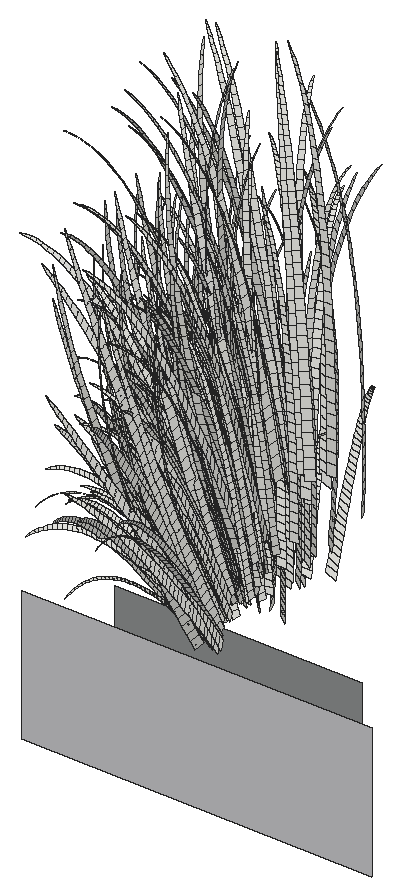
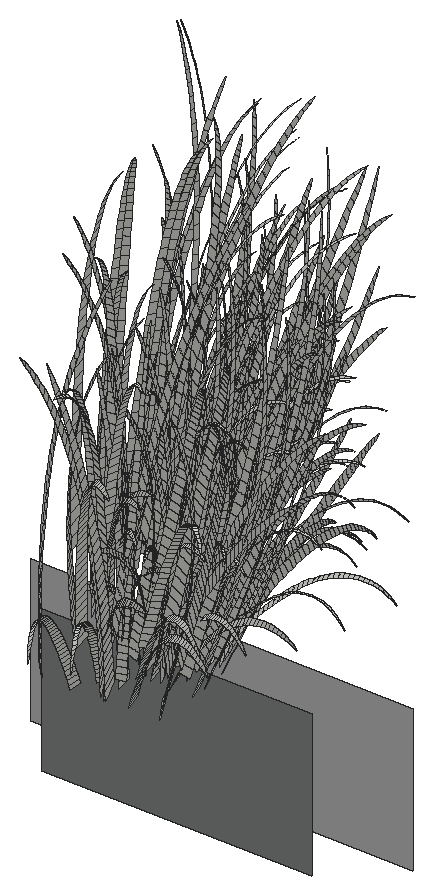
# SketchUp Ruby script. Lengths in inches.
U = 1.inch
M = Sketchup.active_model
def pt(a) = Geom::Point3d.new(a.map { |v| v * U })
def face(e, loops, mat)
  f = e.add_face(loops[0].map { |a| pt(a) })
  loops[1..].each { |l| e.add_face(l.map { |a| pt(a) }).erase! }
  f.material = f.back_material = mat if mat
  f
end
# faces: each face lists its corners as indices into pts; further lists are holes
def faces(e, pts, list, mat = nil) = list.each { |f| face(e, (f[0].is_a?(Array) ? f : [f]).map { |l| l.map { |i| pts[i] } }, mat) }
# xy, xz, yz: faces in a plane at the given z, y or x. An outline is a flat list of corners, or four numbers for a rectangle; further outlines are holes
def ring(l) = l.size == 4 ? [[l[0], l[1]], [l[2], l[1]], [l[2], l[3]], [l[0], l[3]]] : l.each_slice(2).to_a
def flat(e, list, mat, &to3) = list.each { |f| face(e, (f[0].is_a?(Array) ? f : [f]).map { |l| ring(l).map { |u, v| to3.(u, v) } }, mat) }
def xy(e, z, list, mat = nil) = flat(e, list, mat) { |x, y| [x, y, z] }
def xz(e, y, list, mat = nil) = flat(e, list, mat) { |x, z| [x, y, z] }
def yz(e, x, list, mat = nil) = flat(e, list, mat) { |y, z| [x, y, z] }
def lines(e, pts, list) = list.each { |a, b| e.add_line(pt(pts[a]), pt(pts[b])) }
# prism: a flat outline (further loops are holes) pulled along v
def prism(e, loops, v, mat = nil)
  f = face(e, loops, mat); d = Geom::Vector3d.new(v.map { |x| x * U })
  f.pushpull(f.normal.samedirection?(d) ? d.length : -d.length)
end
def box(e, o, s, mat = nil) = prism(e, [[o, [o[0] + s[0], o[1], o[2]], [o[0] + s[0], o[1] + s[1], o[2]], [o[0], o[1] + s[1], o[2]]]], [0, 0, s[2]], mat)
def at(x, y, z, deg = 0) = Geom::Transformation.translation(pt([x, y, z])) * Geom::Transformation.rotation(ORIGIN, Z_AXIS, deg.degrees)
def axes(o, x, y, z) = Geom::Transformation.new([*x, 0, *y, 0, *z, 0, *pt(o).to_a, 1])
def part(name) = M.definitions.add(name)
# library, detail: a bought-in or finely detailed component or shape, given as its bounding box
def library(name, o, s) = part(name).tap { |d| box(d.entities, o, s) }
def detail(e, o, s) = box(e.add_group.entities, o, s)
def put(e, d, t, mat = nil) = e.add_instance(d, t).tap { |i| i.material = mat if mat }
def group(e, t, mat = nil) = e.add_group.tap { |g| g.transformation = t; g.material = mat if mat }.entities
root = M.entities
M.materials.add("[Blacktop Old 02]").color = [143, 145, 145]
M.materials.add("[Polished Concrete New]").color = [200, 200, 203]
c1 = part("fur_instance\#8")
p = [[-0.25,1.49,0.03],[0.25,-1.49,-0.03],[0.44,-1.47,1.51],[-0.05,1.47,1.57],[0.65,-1.44,3.05],[0.16,1.45,3.11],
  [0.86,-1.42,4.59],[0.38,1.44,4.65],[1.1,-1.39,6.13],[0.62,1.43,6.18],[1.34,-1.35,7.66],[0.875,1.42,7.72],
  [1.6,-1.32,9.19],[1.14,1.41,9.25],[1.88,-1.28,10.72],[1.43,1.41,10.78],[2.18,-1.24,12.25],[1.73,1.41,12.3],
  [2.49,-1.19,13.77],[2.05,1.41,13.82],[2.83,-1.15,15.29],[2.4,1.41,15.34],[3.18,-1.09,16.8],[2.76,1.42,16.85],
  [3.56,-1.03,18.31],[3.14,1.43,18.35],[3.96,-0.97,19.81],[3.55,1.44,19.85],[4.38,-0.91,21.3],[3.99,1.46,21.35],
  [4.84,-0.83,22.78],[4.45,1.48,22.83],[5.32,-0.76,24.26],[4.93,1.51,24.31],[5.82,-0.67,25.73],[5.45,1.54,25.77],
  [6.36,-0.59,27.18],[6,1.57,27.23],[6.93,-0.49,28.625],[6.58,1.61,28.67],[7.54,-0.39,30.05],[7.19,1.66,30.1],
  [8.18,-0.28,31.47],[7.84,1.71,31.51],[8.85,-0.16,32.86],[8.53,1.77,32.9],[9.57,-0.04,34.24],[9.25,1.83,34.27],
  [10.32,0.09,35.59],[10.02,1.9,35.625],[11.12,0.23,36.92],[10.82,1.97,36.95],[11.95,0.38,38.22],[11.67,2.06,38.25],
  [12.84,0.54,39.49],[12.57,2.14,39.52],[13.76,0.71,40.73],[13.51,2.24,40.76],[14.73,0.89,41.93],[14.49,2.34,41.95],
  [15.75,1.08,43.09],[15.52,2.45,43.11],[16.82,1.28,44.2],[16.6,2.5625,44.23],[17.93,1.5,45.27],[17.73,2.68,45.29],
  [19.08,1.73,46.28],[18.9,2.81,46.3],[20.29,1.97,47.24],[20.125,2.93,47.26],[21.53,2.22,48.13],[21.39,3.0625,48.15],
  [22.82,2.5,48.96],[22.7,3.1875,48.98],[24.14,2.8125,49.72],[24.06,3.3,49.73],[25.48,3.27,50.41]]
faces(c1.entities,p,[[0,1,2,3],[3,2,4,5],[5,4,6,7],[7,6,8,9],[9,8,10,11],[11,10,12,13],[13,12,14,15],[15,14,16,17],
  [17,16,18,19],[19,18,20,21],[21,20,22,23],[23,22,24,25],[25,24,26,27],[27,26,28,29],[29,28,30,31],[31,30,32,33],
  [33,32,34,35],[35,34,36,37],[37,36,38,39],[39,38,40,41],[41,40,42,43],[43,42,44,45],[45,44,46,47],[47,46,48,49],
  [49,48,50,51],[51,50,52,53],[53,52,54,55],[55,54,56,57],[57,56,58,59],[59,58,60,61],[61,60,62,63],[63,62,64,65],
  [65,64,66,67],[67,66,68,69],[69,68,70,71],[71,70,72,73],[73,72,74,75],[75,74,76]])
xz(root,47.02,[[415.52,0,442.8125,10.375]],"[Polished Concrete New]")
xz(root,51.02,[[419.51,0,438.8125,10.375]],"[Blacktop Old 02]")
put(root,c1,axes([426.79,51.39,16.74],[-0.23554,0.05296,-0.19778],[0.0198,-0.2043,-0.19606],[-0.09324,-0.11985,0.49597]))
put(root,c1,axes([425.38,56.38,16.61],[-0.04995,0.23864,-0.11124],[-0.21419,-0.02204,-0.24055],[-0.12191,-0.01612,0.49664]))
put(root,c1,axes([426.6,51.125,11.45],[-0.11039,-0.00414,-0.3495],[0.07669,-0.1786,0.00651],[-0.14786,-0.06719,0.2791]))
put(root,c1,axes([427.18,49.875,11.47],[-0.13594,0.15084,-0.11164],[-0.0609,-0.07291,-0.33491],[-0.13519,-0.09407,0.27953]))
put(root,c1,axes([426.68,55.02,12.58],[-0.1218,-0.13361,-0.0921],[0.11484,-0.14709,0.28095],[-0.12602,0.02393,0.36414]))
put(root,c1,axes([427.19,53.87,10.88],[-0.1289,0.01316,-0.29885],[-0.02366,-0.17656,0.13341],[-0.13753,0.03975,0.27153]))
put(root,c1,axes([424.89,53.64,11.67],[0.13391,-0.00422,0.37894],[-0.02725,0.21287,-0.08205],[-0.17659,-0.01268,0.31548]))
put(root,c1,axes([426.69,57.03,14.76],[-0.09952,0.18231,-0.31022],[-0.16857,-0.11721,-0.10121],[-0.1255,0.04853,0.40556]))
put(root,c1,axes([424.78,54.78,11.59],[0.14067,-0.04522,0.3848],[0.02544,0.20918,-0.05629],[-0.17357,0.01812,0.31957]))
put(root,c1,axes([425.36,55.57,13.76],[0.05993,0.19956,0.02934],[-0.16765,0.09615,-0.32784],[-0.14862,0.00196,0.40149]))
put(root,c1,axes([426.36,56.78,16.92],[-0.0789,0.22714,-0.18379],[-0.20548,-0.06456,-0.18143],[-0.11262,0.00359,0.48952]))
put(root,c1,axes([427.34,57.21,11.14],[-0.14657,0.06865,-0.32949],[-0.09952,-0.16829,0.15169],[-0.11649,0.08935,0.30613]))
put(root,c1,axes([427.57,50.6,12.74],[-0.14992,0.10635,-0.20855],[-0.03569,-0.13875,-0.18978],[-0.12006,-0.06524,0.33426]))
put(root,c1,axes([427.57,52.03,12.61],[-0.13947,0.07457,-0.26376],[-0.03048,-0.16347,-0.05841],[-0.12421,-0.01975,0.3263]))
put(root,c1,axes([427.6,50.76,11.21],[-0.11214,0.07357,-0.29467],[-0.00419,-0.1506,-0.10442],[-0.13991,-0.03543,0.25192]))
put(root,c1,axes([426.66,54.32,19.19],[-0.16722,-0.14584,-0.14657],[0.18274,-0.19209,0.09427],[-0.0816,-0.06233,0.55718]))
put(root,c1,axes([427.44,54.59,11.82],[-0.12578,-0.12091,-0.0564],[0.08033,-0.12818,0.33188],[-0.12725,0.06361,0.28183]))
put(root,c1,axes([427.75,56.86,19.51],[-0.24661,-0.01011,-0.12308],[0.03558,-0.24626,0.10561],[-0.06805,-0.01098,0.55498]))
put(root,c1,axes([425.25,57.28,11.43],[0.15352,0.06911,0.26676],[-0.03494,0.20117,-0.28887],[-0.16523,0.04776,0.32623]))
put(root,c1,axes([425.19,55.28,12.72],[0.10956,-0.18152,0.25882],[0.13509,0.11782,0.19082],[-0.14519,0.00192,0.39222]))
put(root,c1,axes([426.18,53.23,12.1],[0.07012,-0.18381,0.20265],[0.10518,0.07075,0.29594],[-0.16336,-0.01173,0.29184]))
put(root,c1,axes([426.59,53.01,16.52],[-0.04128,-0.19919,-0.10991],[0.2038,-0.09544,0.23105],[-0.11682,-0.05581,0.46862]))
put(root,c1,axes([427.86,55.84,12.125],[-0.12441,0.08913,-0.33358],[-0.11522,-0.1494,0.09624],[-0.1115,0.08552,0.29301]))
put(root,c1,axes([425.76,51.14,10.98],[0.13283,-0.0342,0.36955],[-0.05695,0.18902,0.06859],[-0.15898,-0.07225,0.3001]))
put(root,c1,axes([426.07,51.01,11.44],[0.11177,0.01694,0.37048],[-0.08915,0.18926,-0.03147],[-0.15727,-0.07147,0.29687]))
put(root,c1,axes([426.59,51.64,11.96],[0.07273,0.09595,0.27862],[-0.10249,0.16133,-0.212],[-0.15668,-0.03967,0.28211]))
put(root,c1,axes([425.11,52.54,12.71],[0.16226,-0.13696,0.26442],[0.06401,0.16282,0.19515],[-0.14822,-0.05035,0.39313]))
put(root,c1,axes([427.95,52.64,17.74],[-0.19486,-0.07064,-0.15993],[0.11436,-0.20339,0.01183],[-0.07048,-0.06892,0.50496]))
put(root,c1,axes([427.38,58.9,16.65],[-0.12046,-0.19753,0.07695],[0.20061,-0.12871,0.24478],[-0.08711,0.03599,0.49657]))
put(root,c1,axes([428.29,55.15,15.83],[-0.16212,0.13096,-0.2268],[-0.11678,-0.16208,0.00347],[-0.08971,0.01858,0.43465]))
put(root,c1,axes([428.23,53.08,11.33],[-0.11086,0.06293,-0.29386],[-0.07533,-0.1452,0.07106],[-0.11428,0.05713,0.25311]))
put(root,c1,axes([428.16,49.42,10.79],[-0.09839,0.14314,-0.01192],[-0.08354,-0.02419,-0.30566],[-0.11714,-0.08151,0.24221]))
put(root,c1,axes([427.55,52.27,11.29],[-0.01321,-0.17005,0.06481],[0.1141,-0.02557,0.30569],[-0.13946,0.01456,0.25678]))
put(root,c1,axes([428.66,53.23,15.55],[-0.18243,0.01895,-0.19563],[-0.00133,-0.1948,0.08688],[-0.09334,0.00298,0.40574]))
put(root,c1,axes([428.14,60.79,16.22],[-0.18658,0.14503,-0.30144],[-0.1645,-0.17028,0.18908],[-0.06369,0.10062,0.4514]))
put(root,c1,axes([428.72,48.89,11.48],[-0.12873,0.10197,-0.18861],[-0.01018,-0.10343,-0.24101],[-0.11719,-0.08155,0.24232]))
put(root,c1,axes([428.53,51.95,13.6],[-0.16023,0.03354,-0.19126],[-0.00898,-0.17162,0.02853],[-0.08895,-0.01176,0.36236]))
put(root,c1,axes([428.06,52.97,12.5],[-0.0676,0.15738,-0.2157],[-0.13135,-0.07732,-0.14677],[-0.1112,0.02111,0.32133]))
put(root,c1,axes([428.49,50.69,14.9375],[-0.1494,0.14445,-0.05993],[-0.10862,-0.10225,-0.21391],[-0.08642,-0.08137,0.39881]))
put(root,c1,axes([425.98,52.1875,13.6],[0.16036,-0.12824,0.26431],[0.05712,0.1633,0.18167],[-0.14465,-0.04914,0.38366]))
put(root,c1,axes([428,52.12,15.66],[-0.08516,-0.14739,-0.15062],[0.16457,-0.13044,0.17116],[-0.1041,-0.04973,0.41758]))
put(root,c1,axes([426.39,52.24,12.83],[0.12489,0.06673,0.27563],[-0.09958,0.18305,-0.12082],[-0.13573,-0.04611,0.36]))
put(root,c1,axes([428.82,48.28,11.89],[-0.15935,0.03269,-0.28558],[0.09029,-0.13292,-0.22683],[-0.09601,-0.14239,0.28508]))
put(root,c1,axes([428.82,48.72,11.18],[-0.14081,0.09765,-0.1356],[-0.01218,-0.08683,-0.27326],[-0.10036,-0.10168,0.23982]))
put(root,c1,axes([428.96,50.15,15.48],[-0.18347,0.1171,-0.07334],[-0.07461,-0.13251,-0.22152],[-0.07812,-0.10043,0.41558]))
put(root,c1,axes([428.84,48.58,11.68],[-0.15082,0.11254,-0.07354],[-0.05779,-0.09193,-0.25822],[-0.08893,-0.09949,0.31347]))
put(root,c1,axes([428.79,50.79,13.44],[-0.15052,-0.00251,-0.18515],[0.03159,-0.16716,0.03488],[-0.08794,-0.02622,0.34898]))
put(root,c1,axes([428.83,50.58,14.92],[-0.149,-0.04647,-0.21352],[0.09287,-0.17245,0.02054],[-0.09229,-0.06322,0.38876]))
put(root,c1,axes([428.96,53.85,16.78],[-0.20159,0.0718,-0.13723],[-0.04865,-0.19336,0.01671],[-0.06325,-0.01861,0.46524]))
put(root,c1,axes([428.85,53.46,11.04],[-0.13656,-0.07352,-0.06681],[0.04427,-0.12761,0.28622],[-0.09439,0.0724,0.24805]))
put(root,c1,axes([428.77,58.21,17.75],[-0.1589,0.17803,-0.2479],[-0.17756,-0.14881,0.0508],[-0.06832,0.04712,0.49383]))
put(root,c1,axes([428.87,52.13,12],[-0.10384,0.1021,-0.23208],[-0.0841,-0.12138,-0.04288],[-0.10059,0.0191,0.29067]))
put(root,c1,axes([428.34,48.34,12.01],[-0.09966,0.12678,0.30336],[-0.19172,0.0268,-0.26785],[-0.07616,-0.17634,0.31506]))
put(root,c1,axes([428.51,52.76,14.16],[-0.10618,-0.13262,-0.04878],[0.13367,-0.1263,0.19427],[-0.08735,0.00279,0.37967]))
put(root,c1,axes([428.99,57.38,11.26],[-0.17971,0.05049,-0.21333],[-0.08082,-0.15328,0.27859],[-0.06056,0.11282,0.29972]))
put(root,c1,axes([427.36,52.25,10.78],[0.10833,0.05099,0.24664],[-0.03776,0.16401,-0.19126],[-0.1393,0.01454,0.25647]))
put(root,c1,axes([428.48,54.85,20.375],[-0.09372,-0.20637,-0.07363],[0.22677,-0.12712,0.15354],[-0.08199,-0.04812,0.55353]))
put(root,c1,axes([427.59,50.48,12.19],[0.05365,-0.16969,-0.03778],[0.13986,-0.00916,0.27148],[-0.1167,-0.06341,0.32492]))
put(root,c1,axes([429.32,53.85,12.44],[-0.13323,0.08202,-0.23675],[-0.08835,-0.14174,0.08371],[-0.08237,0.05187,0.31467]))
put(root,c1,axes([429.05,48.83,11.85],[-0.10552,0.13111,0.03774],[-0.1075,-0.03434,-0.24755],[-0.08294,-0.09279,0.29236]))
put(root,c1,axes([429.6,48.91,15.38],[-0.23362,0.09843,0.07428],[-0.08627,-0.11761,-0.36241],[-0.04076,-0.18596,0.42692]))
put(root,c1,axes([428.79,49.16,11.5625],[-0.05906,0.14196,0.06951],[-0.12604,0.00717,-0.23329],[-0.09379,-0.07416,0.28621]))
put(root,c1,axes([426.9,53.26,13.26],[0.15491,-0.05585,0.29054],[0.02871,0.18789,-0.02061],[-0.13151,0.00174,0.35528]))
put(root,c1,axes([429.51,51.98,14.7],[-0.13836,0.10656,-0.19014],[-0.08729,-0.13946,-0.02631],[-0.08371,0.00267,0.36384]))
put(root,c1,axes([427.49,49.11,10.74],[0.08197,-0.14846,-0.17255],[0.1435,-0.03613,0.3122],[-0.11735,-0.1189,0.28043]))
put(root,c1,axes([429.62,51.47,18.39],[-0.2227,-0.02851,-0.13015],[0.07795,-0.20389,-0.10631],[-0.04666,-0.10194,0.51151]))
put(root,c1,axes([428.39,50.93,12.49],[0.03066,0.14936,0.05869],[-0.12804,0.07175,-0.24213],[-0.11455,-0.01821,0.30092]))
put(root,c1,axes([429.01,49.93,11.92],[-0.05395,-0.10392,-0.15053],[0.10796,-0.10426,0.17042],[-0.10255,-0.03484,0.272]))
put(root,c1,axes([428.76,51,16.38],[-0.03053,0.18634,0.11663],[-0.19498,0.03215,-0.20672],[-0.09234,-0.08694,0.42611]))
put(root,c1,axes([428.01,56.42,13.39],[0.01665,-0.19186,0.25247],[0.18867,0.0288,0.15737],[-0.09759,0.06145,0.3728]))
put(root,c1,axes([429.6,48.2,12.62],[-0.17727,0.00029,-0.20455],[0.08516,-0.1353,-0.21935],[-0.05731,-0.14134,0.34686]))
put(root,c1,axes([429.36,48.68,12.49],[-0.10062,-0.049,-0.26041],[0.12035,-0.13237,-0.01381],[-0.08638,-0.09663,0.30447]))
put(root,c1,axes([429.01,50.15,14.97],[-0.076,0.1669,0.09562],[-0.17144,-0.01335,-0.19918],[-0.07397,-0.09509,0.39348]))
put(root,c1,axes([429.47,55.02,20.71],[-0.19599,0.17659,-0.04249],[-0.16606,-0.16516,-0.03794],[-0.03174,-0.0516,0.57661]))
put(root,c1,axes([429.33,51.97,15.31],[-0.14595,-0.08896,-0.08701],[0.11069,-0.159,0.08949],[-0.05969,-0.02587,0.41282]))
put(root,c1,axes([429.33,50.94,15.48],[-0.13003,0.1505,-0.04051],[-0.13515,-0.09639,-0.12681],[-0.0585,-0.05721,0.41915]))
put(root,c1,axes([428.24,53.16,19.38],[-0.01349,0.22403,0.09768],[-0.24396,0.034,-0.14422],[-0.06912,-0.0865,0.54108]))
put(root,c1,axes([429.66,50.28,13.09],[-0.12457,-0.03797,-0.15408],[0.05979,-0.14532,0.07008],[-0.07901,-0.02356,0.31353]))
put(root,c1,axes([429.48,55.42,20.55],[-0.19695,0.1732,-0.04859],[-0.16287,-0.16855,-0.01576],[-0.02749,-0.04327,0.57313]))
put(root,c1,axes([429.3,48.07,13.0625],[-0.15374,0.14658,0.25603],[-0.19784,-0.04817,-0.27014],[-0.04101,-0.18709,0.42951]))
put(root,c1,axes([429.32,53.8,19.28],[-0.20007,-0.1011,-0.05198],[0.13259,-0.20105,0.02025],[-0.03025,-0.05245,0.53866]))
put(root,c1,axes([427.7,49.47,10.74],[0.13307,-0.06357,0.27984],[-0.03809,0.14212,0.17121],[-0.12562,-0.08741,0.25976]))
put(root,c1,axes([429.82,53.67,20.4],[-0.23914,-0.05106,-0.06078],[0.08551,-0.22855,-0.0252],[-0.02809,-0.06875,0.5682]))
put(root,c1,axes([427.47,54.33,16.17],[0.12687,0.1431,0.11306],[-0.15006,0.15928,-0.20805],[-0.10892,-0.0144,0.44372]))
put(root,c1,axes([428.26,52,10.79],[0.06974,-0.11239,0.27242],[0.09117,0.10684,0.0892],[-0.12045,0.03482,0.23783]))
put(root,c1,axes([427.44,53.55,12.375],[0.12819,-0.10555,0.27193],[0.08655,0.15023,0.02614],[-0.11644,0.02211,0.33646]))
put(root,c1,axes([426.89,55.5,13.38],[0.17949,0.03208,0.20009],[-0.02216,0.19765,-0.22548],[-0.11594,0.04484,0.37468]))
put(root,c1,axes([428.58,54.41,15.93],[0.00664,0.20286,-0.1262],[-0.19518,0.01818,-0.18229],[-0.08769,0.01816,0.42485]))
put(root,c1,axes([429.57,48.37,11.35],[-0.0986,0.1202,0.03133],[-0.09749,-0.03341,-0.22837],[-0.07635,-0.08541,0.26912]))
put(root,c1,axes([430.06,56.61,13.21],[-0.18808,0.05687,-0.16759],[-0.06647,-0.17012,0.23097],[-0.05108,0.08069,0.36201]))
put(root,c1,axes([429.36,48.13,10.95],[-0.08725,-0.02366,-0.29756],[0.12591,-0.11202,-0.06714],[-0.0803,-0.1191,0.23844]))
put(root,c1,axes([429.89,48.21,11.93],[-0.15103,0.03829,-0.1475],[0.02836,-0.11444,-0.19385],[-0.06472,-0.10394,0.28282]))
put(root,c1,axes([427.19,49.96,12.54],[0.17403,-0.06722,0.24815],[-0.01797,0.16553,0.179],[-0.11789,-0.09322,0.35975]))
put(root,c1,axes([428.86,47.625,10.93],[-0.07738,0.12181,0.42116],[-0.24475,0.02807,-0.19007],[-0.04925,-0.2161,0.35893]))
put(root,c1,axes([427.55,55.9375,13.65],[0.149,0.11824,0.07488],[-0.1012,0.16059,-0.29075],[-0.11547,0.04466,0.37315]))
put(root,c1,axes([430.08,47.65,11.93],[-0.19758,0.0885,0.1271],[-0.09447,-0.05952,-0.37318],[-0.04202,-0.18438,0.30623]))
put(root,c1,axes([428.43,50.7,11.09],[0.09888,-0.02928,0.28041],[-0.00291,0.15131,-0.01175],[-0.12783,-0.00918,0.22836]))
put(root,c1,axes([428.21,57.21,12.21],[0.03058,-0.16302,0.35291],[0.18885,0.05742,0.07777],[-0.09099,0.10522,0.30707]))
put(root,c1,axes([428.5625,49.52,12.4],[0.04667,0.10587,0.22641],[-0.14224,0.11026,-0.13144],[-0.10087,-0.07976,0.30781]))
put(root,c1,axes([428.95,52.48,12.72],[-0.01787,-0.16163,0.13786],[0.14541,-0.01364,0.20157],[-0.09392,0.03632,0.30351]))
put(root,c1,axes([429.45,49.06,15.16],[-0.12023,0.16893,0.15811],[-0.19192,-0.04724,-0.20175],[-0.05017,-0.13536,0.45159]))
put(root,c1,axes([429.875,50.97,14.51],[-0.15295,0.08658,-0.10984],[-0.06653,-0.14152,-0.02919],[-0.05435,-0.02356,0.3759]))
put(root,c1,axes([429.71,48.89,13.5],[-0.1513,-0.02821,-0.17374],[0.08683,-0.1419,-0.10144],[-0.05423,-0.09755,0.35603]))
put(root,c1,axes([427.34,55.62,12.7],[0.1591,-0.07433,0.27972],[0.07325,0.17912,-0.08368],[-0.11229,0.04342,0.36287]))
put(root,c1,axes([430.02,55.96,14.02],[-0.16185,0.10098,-0.22361],[-0.11509,-0.14728,0.17524],[-0.05085,0.08033,0.3604]))
put(root,c1,axes([429.53,52.42,12.74],[-0.08732,-0.12975,0.07004],[0.12156,-0.08169,0.22443],[-0.07712,0.04857,0.29461]))
put(root,c1,axes([428.11,54.28,11.23],[0.12181,-0.05572,0.30355],[0.07119,0.15699,-0.09562],[-0.1203,0.06014,0.26644]))
put(root,c1,axes([430.35,53.54,20.46],[-0.24023,0.10194,-0.01182],[-0.08393,-0.20819,-0.06775],[-0.02132,-0.07588,0.56748]))
put(root,c1,axes([429.83,48.68,12.42],[-0.07947,0.12548,0.07397],[-0.11521,-0.01055,-0.22059],[-0.07706,-0.08621,0.27164]))
put(root,c1,axes([428.07,51.02,12.4375],[0.13512,-0.04534,0.25565],[0.00767,0.16418,0.01521],[-0.11775,-0.01872,0.30933]))
put(root,c1,axes([430.23,50.95,14.47],[-0.16155,0.04363,-0.11105],[-0.02173,-0.15615,0.00187],[-0.05311,-0.02302,0.36735]))
put(root,c1,axes([428.15,54.34,11.75],[0.14298,0.02776,0.2221],[0.00324,0.16655,-0.23396],[-0.12194,0.06096,0.27007]))
put(root,c1,axes([429.54,50.91,12.84],[-0.06439,-0.12354,-0.04587],[0.12333,-0.08786,0.16125],[-0.07712,-0.0102,0.31415]))
put(root,c1,axes([430.14,52.2,14.37],[-0.13763,-0.08778,-0.02445],[0.09224,-0.14199,0.18002],[-0.06167,0.02548,0.35158]))
put(root,c1,axes([428.99,49.17,11.46],[0.02731,-0.14018,-0.06519],[0.12315,-0.02871,0.2214],[-0.09827,-0.0534,0.27359]))
put(root,c1,axes([430.23,61.88,14.33],[-0.20442,-0.12057,0.16665],[0.14603,-0.18202,0.30806],[-0.03237,0.10426,0.44592]))
put(root,c1,axes([428.38,48.72,10.87],[0.09631,-0.13966,-0.10726],[0.11682,-0.00954,0.30869],[-0.10751,-0.10893,0.25692]))
put(root,c1,axes([430.3125,48.8,14.07],[-0.18173,0.02045,-0.09763],[0.0261,-0.14072,-0.18343],[-0.04068,-0.10974,0.36609]))
put(root,c1,axes([429.46,57.31,11.78],[-0.05838,0.1486,-0.35065],[-0.18856,-0.06365,0.02437],[-0.06066,0.11302,0.30025]))
put(root,c1,axes([428.79,49.96,12.25],[0.06905,-0.15041,0.07394],[0.1069,0.0384,0.22809],[-0.10814,-0.03674,0.28683]))
put(root,c1,axes([429.83,51.97,18.8],[-0.11071,0.19643,0.08485],[-0.20741,-0.05916,-0.14436],[-0.04649,-0.10158,0.50968]))
put(root,c1,axes([430.01,54.9,12.82],[-0.12886,0.11444,-0.22997],[-0.12949,-0.11784,0.12414],[-0.04678,0.07389,0.33152]))
put(root,c1,axes([428.76,50.34,13.82],[0.02994,-0.16585,-0.05499],[0.16129,-0.01842,0.19273],[-0.08623,-0.05907,0.36324]))
put(root,c1,axes([428.15,51.4375,14.73],[0.12398,0.09622,0.18511],[-0.12468,0.16008,-0.11198],[-0.09878,-0.04719,0.39625]))
put(root,c1,axes([430.4,47.57,11.5],[-0.18497,0.04944,-0.02341],[-0.00878,-0.07542,-0.33252],[-0.03553,-0.1559,0.25894]))
put(root,c1,axes([430.12,49.82,14.43],[-0.14413,-0.05167,-0.11933],[0.08701,-0.14734,-0.01287],[-0.04763,-0.0596,0.37283]))
put(root,c1,axes([429.83,47.92,11.125],[-0.04193,0.09854,0.23039],[-0.14173,0.04993,-0.18317],[-0.07748,-0.11492,0.23007]))
put(root,c1,axes([428.5,58.4,16.19],[0.04781,0.21803,-0.18144],[-0.22564,0.05394,-0.16456],[-0.06613,0.04562,0.47803]))
put(root,c1,axes([430.47,51.35,15.28],[-0.15275,-0.06369,-0.07605],[0.08272,-0.1606,0.08732],[-0.05298,-0.01559,0.38969]))
put(root,c1,axes([427.3,59.35,12.77],[0.19488,-0.04118,0.27862],[0.0814,0.18631,-0.28554],[-0.10045,0.11615,0.33899]))
put(root,c1,axes([430.3,50.51,14.45],[-0.12167,0.12231,-0.08026],[-0.10576,-0.10199,-0.07795],[-0.05387,-0.03162,0.36369]))
put(root,c1,axes([429.6,50.11,13.17],[-0.02354,-0.13666,-0.06934],[0.13862,-0.06024,0.1585],[-0.07899,-0.03774,0.31687]))
put(root,c1,axes([430.56,47.6875,11.5625],[-0.15528,0.03655,-0.09389],[0.01601,-0.10098,-0.21878],[-0.04549,-0.11219,0.27533]))
put(root,c1,axes([430.59,48.53,13.11],[-0.15238,0.03287,-0.097],[0.00948,-0.12228,-0.14695],[-0.04746,-0.08538,0.3116]))
put(root,c1,axes([429.62,52.82,12.13],[-0.00457,0.15131,-0.19037],[-0.14827,-0.01393,-0.13436],[-0.07643,0.04813,0.29198]))
put(root,c1,axes([428.8,51.8,14.87],[0.1073,0.11537,0.13468],[-0.12896,0.14123,-0.15523],[-0.09593,-0.0286,0.38067]))
put(root,c1,axes([429.48,56.8,19.36],[-0.03892,0.23857,-0.13916],[-0.24331,-0.01786,-0.06409],[-0.04532,0.0056,0.5395]))
put(root,c1,axes([430.7,51.05,14.29],[-0.15222,0.06371,-0.10078],[-0.04912,-0.14483,0.02613],[-0.04368,-0.00705,0.35627]))
put(root,c1,axes([428.73,54.41,11.64],[0.12204,0.11956,-0.03437],[-0.09323,0.10261,-0.31254],[-0.10097,0.07745,0.26536]))
put(root,c1,axes([429.83,49.76,13.5625],[-0.02967,-0.13006,-0.11002],[0.14258,-0.07093,0.13984],[-0.07655,-0.05244,0.32247]))
put(root,c1,axes([430.62,55.04,12.58],[-0.18524,0.01318,-0.044],[-0.00864,-0.16062,0.25477],[-0.0239,0.07696,0.32915]))
put(root,c1,axes([428.71,49.07,11.92],[0.10962,-0.14134,0.02858],[0.09848,0.05163,0.25611],[-0.09929,-0.07851,0.30299]))
put(root,c1,axes([430.2,49.09,14.28],[-0.07622,0.14548,0.11566],[-0.15943,-0.01772,-0.1678],[-0.05494,-0.09882,0.36066]))
put(root,c1,axes([430.2,53.96,14.1875],[-0.11141,0.14453,-0.18255],[-0.14786,-0.09923,0.0582],[-0.03635,0.0417,0.37637]))
put(root,c1,axes([427.29,58.14,16.05],[0.21224,0.07306,0.08848],[-0.08036,0.21667,-0.23259],[-0.08448,0.0349,0.48158]))
put(root,c1,axes([430.93,49.75,17.04],[-0.23536,0.00031,-0.04255],[0.03502,-0.16941,-0.26023],[-0.00865,-0.15175,0.46324]))
put(root,c1,axes([430.91,53.2,11.09],[-0.14803,0.01323,-0.11537],[-0.03176,-0.12328,0.24366],[-0.04653,0.08668,0.23028]))
put(root,c1,axes([429.3,47.98,11.03],[0.07176,0.04443,0.32956],[-0.1495,0.11571,0.02095],[-0.08693,-0.12893,0.25813]))
put(root,c1,axes([430.45,51.98,17.77],[-0.16552,-0.11118,-0.05649],[0.14207,-0.16762,-0.00154],[-0.02412,-0.05905,0.48802]))
put(root,c1,axes([430.41,47.75,12.37],[-0.1192,0.12425,0.22535],[-0.17166,-0.03356,-0.21354],[-0.0342,-0.15606,0.35826]))
put(root,c1,axes([427.29,59.98,13.35],[0.22314,0.03503,0.11397],[-0.0252,0.21097,-0.3146],[-0.08653,0.08429,0.4222]))
put(root,c1,axes([430.85,50.63,16.12],[-0.18454,0.07316,-0.01839],[-0.05778,-0.16138,-0.04792],[-0.01906,-0.05522,0.43193]))
put(root,c1,axes([430.12,49.52,13.59],[-0.02927,-0.12714,-0.10789],[0.13946,-0.06963,0.13664],[-0.0749,-0.05131,0.31553]))
put(root,c1,axes([430.61,55.86,18.2],[-0.15948,0.17543,-0.11844],[-0.17074,-0.13846,0.07646],[-0.0175,0.01182,0.50519]))
put(root,c1,axes([429.55,55.625,19.05],[-0.03022,-0.22611,0.09029],[0.23429,-0.05028,0.11994],[-0.05481,-0.00145,0.5217]))
put(root,c1,axes([428.37,48.91,13.15],[0.13498,-0.15634,-0.12045],[0.15269,0.03421,0.29976],[-0.08583,-0.13785,0.37509]))
put(root,c1,axes([429.04,49.97,15.18],[0.08886,0.11953,0.22309],[-0.17307,0.12603,-0.0526],[-0.07674,-0.09865,0.40821]))
put(root,c1,axes([430.67,52.2,13.18],[-0.10713,0.11469,-0.16211],[-0.11423,-0.10051,0.03718],[-0.0449,0.03097,0.32456]))
put(root,c1,axes([430.96,53.76,19.59],[-0.19122,-0.11806,-0.01455],[0.14538,-0.19433,0.04316],[-0.02276,-0.03764,0.53822]))
put(root,c1,axes([429.97,52.83,15.77],[-0.07059,-0.16734,0.04684],[0.17777,-0.08469,0.11217],[-0.04438,-0.00118,0.42241]))
put(root,c1,axes([429.61,50.14,16.91],[-0.00008,0.17023,0.2439],[-0.22913,0.05018,-0.08813],[-0.05076,-0.13695,0.4569]))
put(root,c1,axes([429.95,57.07,17.09],[-0.03105,0.21618,-0.23248],[-0.22713,-0.0199,-0.04743],[-0.04502,0.05164,0.46606]))
put(root,c1,axes([431.06,51.47,15.15],[-0.1632,-0.04584,-0.02491],[0.06111,-0.16287,0.10545],[-0.03205,0.00396,0.38155]))
put(root,c1,axes([430.28,51.84,14.78],[-0.07809,-0.14325,0.0107],[0.15359,-0.09235,0.11164],[-0.04706,-0.00759,0.38378]))
put(root,c1,axes([428.44,50.28,14.47],[0.15632,-0.13539,0.07566],[0.09629,0.11232,0.20743],[-0.0859,-0.08088,0.3964]))
put(root,c1,axes([428.33,47.9375,11.13],[0.17581,0.00429,0.35889],[-0.15371,0.13999,0.25001],[-0.08231,-0.1906,0.34052]))
put(root,c1,axes([430.42,58.49,11.59],[-0.08555,0.15021,-0.34626],[-0.19424,-0.0665,0.11459],[-0.03163,0.1226,0.31264]))
put(root,c1,axes([431.1,57.58,14.1875],[-0.21697,-0.00618,0.04885],[0.02773,-0.18874,0.29817],[-0.00075,0.0894,0.38532]))
put(root,c1,axes([429.52,49.51,15.26],[0.05112,0.14176,0.22694],[-0.19757,0.09246,-0.06236],[-0.06344,-0.11412,0.4165]))
put(root,c1,axes([428.79,56.21,11.35],[0.12897,-0.08882,0.30598],[0.12311,0.13439,-0.14076],[-0.0848,0.09806,0.28618]))
put(root,c1,axes([430.62,55.55,20.11],[-0.12955,0.21354,-0.0433],[-0.21401,-0.10243,0.0018],[-0.01549,-0.03509,0.55942]))
put(root,c1,axes([429.58,51.82,12.99],[0.05338,0.14377,-0.04693],[-0.14103,0.06373,-0.16463],[-0.0677,0.01402,0.32804]))
put(root,c1,axes([429.86,49.52,13.95],[0.0229,-0.1484,-0.09458],[0.15576,-0.02704,0.16403],[-0.07366,-0.06935,0.33993]))
put(root,c1,axes([431.13,52.3,16.05],[-0.18597,0.0618,-0.02273],[-0.04748,-0.17087,0.02426],[-0.01189,-0.02692,0.4292]))
put(root,c1,axes([430.05,52.75,18.4375],[-0.05249,0.21081,0.00883],[-0.2212,-0.0235,-0.05439],[-0.02833,-0.05377,0.50988]))
put(root,c1,axes([430.15,51.08,16.96],[-0.04613,-0.168,-0.12838],[0.20048,-0.07761,0.07112],[-0.05022,-0.08162,0.45074]))
put(root,c1,axes([429.66,51,16.02],[0.01336,-0.18156,-0.05149],[0.1916,-0.02315,0.12623],[-0.05991,-0.05859,0.42926]))
put(root,c1,axes([429.21,49.18,12.29],[0.13306,-0.03251,0.2141],[-0.03468,0.1366,0.1095],[-0.09265,-0.07326,0.28274]))
put(root,c1,axes([430.71,49.36,15.52],[-0.14651,-0.09517,-0.11625],[0.13838,-0.13795,-0.08263],[-0.01824,-0.0963,0.42995]))
put(root,c1,axes([429.4,51.41,12.26],[0.12505,0.02128,0.17693],[-0.02026,0.14885,-0.13694],[-0.09536,0.01811,0.27556]))
put(root,c1,axes([427.51,54.44,19.27],[0.23978,-0.07082,0.15768],[0.03022,0.22441,0.06362],[-0.07961,-0.06081,0.54364]))
put(root,c1,axes([431.43,50.89,17.98],[-0.22374,-0.02944,-0.01516],[0.05551,-0.18692,-0.16154],[0.00543,-0.11272,0.49003]))
put(root,c1,axes([431.55,57.14,19.58],[-0.22966,0.11975,-0.02971],[-0.1055,-0.20961,0.14888],[0.00986,0.00949,0.54546]))
put(root,c1,axes([430.26,52.37,17.41],[-0.04674,0.1979,-0.00041],[-0.20698,-0.02041,-0.04932],[-0.02674,-0.04637,0.47621]))
put(root,c1,axes([431.51,55.45,14.82],[-0.2047,0.01723,0.00593],[-0.00087,-0.18882,0.20676],[-0.00221,0.04782,0.40893]))
put(root,c1,axes([431.18,55.5625,19.78],[-0.15522,0.19417,-0.03161],[-0.19201,-0.12962,0.02598],[-0.00591,-0.03393,0.55136]))
put(root,c1,axes([429.56,53.83,11.1875],[0.10395,0.11836,-0.12851],[-0.11439,0.07411,-0.26217],[-0.07351,0.08501,0.2481]))
put(root,c1,axes([427.92,52.16,18.76],[0.21026,0.07749,0.17035],[-0.13208,0.20951,0.0486],[-0.06062,-0.09852,0.54406]))
put(root,c1,axes([428.27,53.16,16.82],[0.19711,0.03834,0.13931],[-0.07116,0.20343,-0.04176],[-0.07003,-0.0411,0.47276]))
put(root,c1,axes([429.625,51.97,13.61],[0.08378,-0.14307,0.16626],[0.13275,0.07958,0.06416],[-0.07048,0.0146,0.34149]))
put(root,c1,axes([428.37,56.94,16.09],[0.2158,0.0049,0.14651],[-0.01279,0.21776,-0.18636],[-0.08047,0.03325,0.45875]))
put(root,c1,axes([430.33,47.82,12.0625],[-0.00857,-0.10681,-0.26092],[0.17656,-0.05814,0.06779],[-0.05152,-0.12704,0.31177]))
put(root,c1,axes([429.23,48.72,12.71],[0.14194,0.01295,0.23971],[-0.09799,0.13483,0.13149],[-0.07264,-0.11667,0.31745]))
put(root,c1,axes([431.42,49.53,14.31],[-0.14611,0.07417,-0.01085],[-0.0636,-0.12579,-0.04088],[-0.01571,-0.04551,0.35595]))
put(root,c1,axes([430.09,48.25,12.27],[0.04246,-0.11664,-0.17724],[0.14637,-0.02684,0.16417],[-0.06419,-0.10309,0.2805]))
put(root,c1,axes([431.59,53.49,16.57],[-0.17716,0.11278,-0.05906],[-0.10338,-0.15992,0.10796],[-0.00363,0.01008,0.44244]))
